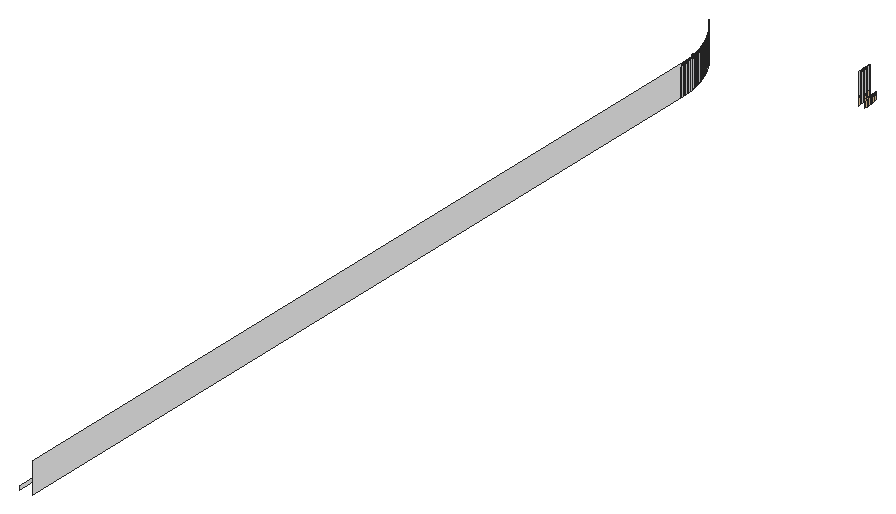
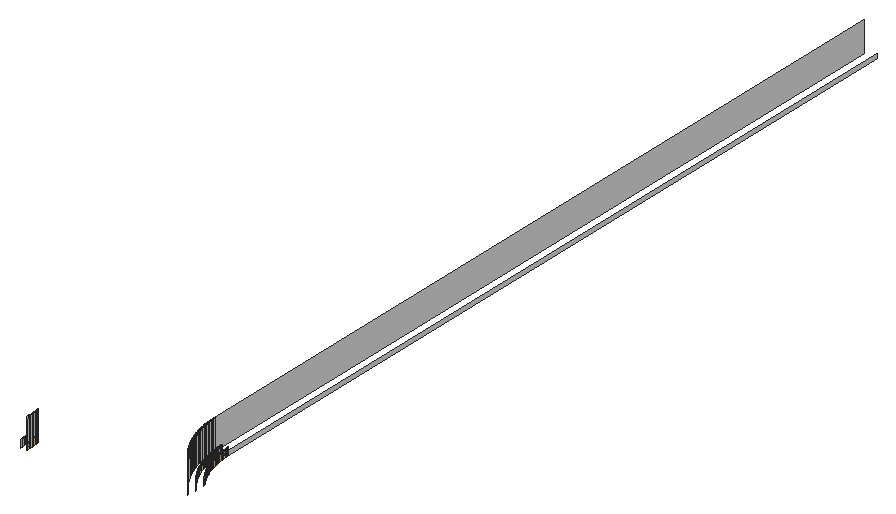
# SketchUp Ruby script. Lengths in inches.
U = 1.inch
M = Sketchup.active_model
def pt(a) = Geom::Point3d.new(a.map { |v| v * U })
def face(e, loops, mat)
  f = e.add_face(loops[0].map { |a| pt(a) })
  loops[1..].each { |l| e.add_face(l.map { |a| pt(a) }).erase! }
  f.material = f.back_material = mat if mat
  f
end
# faces: each face lists its corners as indices into pts; further lists are holes
def faces(e, pts, list, mat = nil) = list.each { |f| face(e, (f[0].is_a?(Array) ? f : [f]).map { |l| l.map { |i| pts[i] } }, mat) }
# xy, xz, yz: faces in a plane at the given z, y or x. An outline is a flat list of corners, or four numbers for a rectangle; further outlines are holes
def ring(l) = l.size == 4 ? [[l[0], l[1]], [l[2], l[1]], [l[2], l[3]], [l[0], l[3]]] : l.each_slice(2).to_a
def flat(e, list, mat, &to3) = list.each { |f| face(e, (f[0].is_a?(Array) ? f : [f]).map { |l| ring(l).map { |u, v| to3.(u, v) } }, mat) }
def xy(e, z, list, mat = nil) = flat(e, list, mat) { |x, y| [x, y, z] }
def xz(e, y, list, mat = nil) = flat(e, list, mat) { |x, z| [x, y, z] }
def yz(e, x, list, mat = nil) = flat(e, list, mat) { |y, z| [x, y, z] }
def lines(e, pts, list) = list.each { |a, b| e.add_line(pt(pts[a]), pt(pts[b])) }
# prism: a flat outline (further loops are holes) pulled along v
def prism(e, loops, v, mat = nil)
  f = face(e, loops, mat); d = Geom::Vector3d.new(v.map { |x| x * U })
  f.pushpull(f.normal.samedirection?(d) ? d.length : -d.length)
end
def box(e, o, s, mat = nil) = prism(e, [[o, [o[0] + s[0], o[1], o[2]], [o[0] + s[0], o[1] + s[1], o[2]], [o[0], o[1] + s[1], o[2]]]], [0, 0, s[2]], mat)
def at(x, y, z, deg = 0) = Geom::Transformation.translation(pt([x, y, z])) * Geom::Transformation.rotation(ORIGIN, Z_AXIS, deg.degrees)
def axes(o, x, y, z) = Geom::Transformation.new([*x, 0, *y, 0, *z, 0, *pt(o).to_a, 1])
def part(name) = M.definitions.add(name)
# library, detail: a bought-in or finely detailed component or shape, given as its bounding box
def library(name, o, s) = part(name).tap { |d| box(d.entities, o, s) }
def detail(e, o, s) = box(e.add_group.entities, o, s)
def put(e, d, t, mat = nil) = e.add_instance(d, t).tap { |i| i.material = mat if mat }
def group(e, t, mat = nil) = e.add_group.tap { |g| g.transformation = t; g.material = mat if mat }.entities
root = M.entities
M.materials.add("False Ceiling Light").color = [254, 223, 179]
M.materials.add("[Quartz Light Grey]").color = [251, 251, 252]
yz(root,178.5,[[204,115.32,204.18,116.49],[204.18,115.32,204.35,116.49]],"False Ceiling Light")
yz(root,178.5,[[78,115.32,204,115.91],[204,115.32,204.18,115.91],[204.18,115.32,204.35,115.91]],"[Quartz Light Grey]")
yz(root,179.5,[[204.01,115.32,204.19,116.49],[204.19,115.32,204.38,116.49]],"False Ceiling Light")
yz(root,180.49,[[204.41,115.32,204.61,120]],"[Quartz Light Grey]")
yz(root,180.5,[[77.99,115.32,204.01,120],[204.01,115.32,204.2,120]],"[Quartz Light Grey]")
yz(root,198.5,[[215.99,115.32,216.23,116.49],[216.23,115.32,216.45,116.49]],"False Ceiling Light")
yz(root,198.5,[[215.99,115.32,216.23,120],[216.23,115.32,216.45,120]],"[Quartz Light Grey]")
yz(root,199.5,[[216,115.32,216.24,116.49],[216.24,115.32,216.47,116.49]],"False Ceiling Light")
p = [[180.49,204.41,115.32],[180.5,204.2,115.32],[180.5,204.2,120],[180.49,204.41,120],[178.49,204.53,115.32],[178.5,204.35,115.32],
  [178.5,204.35,116.49],[178.49,204.53,116.49],[178.5,204.35,115.32],[178.49,204.53,115.32],[178.49,204.53,115.91],[178.5,204.35,115.91],
  [179.5,204.38,115.32],[179.49,204.57,115.32],[179.49,204.57,116.49],[179.5,204.38,116.49],[178.48,204.71,115.32],[178.48,204.71,116.49],
  [178.48,204.71,115.32],[178.48,204.71,115.91],[179.48,204.76,115.32],[179.48,204.76,116.49],[180.48,204.8125,115.32],[180.49,204.61,115.32],
  [180.49,204.61,120],[180.48,204.8125,120],[178.47,204.88,115.32],[178.47,204.88,116.49],[178.47,204.88,115.32],[178.47,204.88,115.91],
  [179.47,204.95,115.32],[179.47,204.95,116.49],[180.47,205.01,115.32],[180.47,205.01,120],[178.46,205.06,115.32],[178.46,205.06,116.49],
  [178.46,205.06,115.32],[178.46,205.06,115.91],[179.46,205.14,115.32],[179.46,205.14,116.49],[180.45,205.22,115.32],[180.45,205.22,120],
  [178.44,205.24,115.32],[178.44,205.24,116.49],[178.44,205.24,115.32],[178.44,205.24,115.91],[179.4375,205.33,115.32],[179.4375,205.33,116.49],
  [178.43,205.41,115.32],[178.43,205.41,116.49],[178.43,205.41,115.32],[178.43,205.41,115.91],[180.44,205.42,115.32],[180.44,205.42,120],
  [179.42,205.52,115.32],[179.42,205.52,116.49],[178.41,205.59,115.32],[178.41,205.59,116.49],[178.41,205.59,115.32],[178.41,205.59,115.91],
  [180.42,205.62,115.32],[180.42,205.62,120],[179.4,205.7,115.32],[179.4,205.7,116.49],[178.38,205.76,115.32],[178.38,205.76,116.49],
  [178.38,205.76,115.32],[178.38,205.76,115.91],[180.39,205.82,115.32],[180.39,205.82,120],[179.375,205.89,115.32],[179.375,205.89,116.49],
  [178.36,205.9375,115.32],[178.36,205.9375,116.49],[178.36,205.9375,115.32],[178.36,205.9375,115.91],[180.37,206.02,115.32],[180.37,206.02,120],
  [178.33,206.11,115.32],[178.33,206.11,116.49],[178.33,206.11,115.32],[178.33,206.11,115.91],[179.35,206.08,115.32],[179.35,206.08,116.49],
  [180.34,206.22,115.32],[180.34,206.22,120],[178.31,206.29,115.32],[178.31,206.29,116.49],[178.31,206.29,115.32],[178.31,206.29,115.91],
  [179.32,206.27,115.32],[179.32,206.27,116.49],[180.31,206.42,115.32],[180.31,206.42,120],[178.27,206.46,115.32],[178.27,206.46,116.49],
  [178.27,206.46,115.32],[178.27,206.46,115.91],[179.29,206.46,115.32],[179.29,206.46,116.49],[180.28,206.625,115.32],[180.28,206.625,120],
  [178.24,206.63,115.32],[178.24,206.63,116.49],[178.24,206.63,115.32],[178.24,206.63,115.91],[179.26,206.64,115.32],[179.26,206.64,116.49],
  [178.21,206.81,115.32],[178.21,206.81,116.49],[178.21,206.81,115.32],[178.21,206.81,115.91],[179.22,206.83,115.32],[179.22,206.83,116.49],
  [180.24,206.82,115.32],[180.24,206.82,120],[178.17,206.98,115.32],[178.17,206.98,116.49],[178.17,206.98,115.32],[178.17,206.98,115.91],
  [179.18,207.01,115.32],[179.18,207.01,116.49],[180.2,207.02,115.32],[180.2,207.02,120],[178.13,207.15,115.32],[178.13,207.15,116.49],
  [178.13,207.15,115.32],[178.13,207.15,115.91],[179.14,207.2,115.32],[179.14,207.2,116.49],[180.16,207.22,115.32],[180.16,207.22,120],
  [178.08,207.32,115.32],[178.08,207.32,116.49],[178.08,207.32,115.32],[178.08,207.32,115.91],[179.1,207.38,115.32],[179.1,207.38,116.49],
  [180.12,207.42,115.32],[180.12,207.42,120],[178.04,207.49,115.32],[178.04,207.49,116.49],[178.04,207.49,115.32],[178.04,207.49,115.91],
  [179.05,207.57,115.32],[179.05,207.57,116.49],[180.07,207.62,115.32],[180.07,207.62,120],[177.99,207.66,115.32],[177.99,207.66,116.49],
  [177.99,207.66,115.32],[177.99,207.66,115.91],[179.01,207.75,115.32],[179.01,207.75,116.49],[180.02,207.82,115.32],[180.02,207.82,120],
  [177.94,207.83,115.32],[177.94,207.83,116.49],[177.94,207.83,115.32],[177.94,207.83,115.91],[177.89,208,115.32],[177.89,208,116.49],
  [177.89,208,115.32],[177.89,208,115.91],[178.96,207.9375,115.32],[178.96,207.9375,116.49],[179.97,208.01,115.32],[179.97,208.01,120],
  [178.9,208.12,115.32],[178.9,208.12,116.49],[177.84,208.17,115.32],[177.84,208.17,116.49],[177.84,208.17,115.32],[177.84,208.17,115.91],
  [179.92,208.21,115.32],[179.92,208.21,120],[178.85,208.3,115.32],[178.85,208.3,116.49],[177.78,208.34,115.32],[177.78,208.34,116.49],
  [177.78,208.34,115.32],[177.78,208.34,115.91],[179.86,208.4,115.32],[179.86,208.4,120],[177.73,208.51,115.32],[177.73,208.51,116.49],
  [177.73,208.51,115.32],[177.73,208.51,115.91],[178.79,208.48,115.32],[178.79,208.48,116.49],[179.8,208.6,115.32],[179.8,208.6,120],
  [177.67,208.67,115.32],[177.67,208.67,116.49],[177.67,208.67,115.32],[177.67,208.67,115.91],[178.73,208.66,115.32],[178.73,208.66,116.49],
  [179.74,208.79,115.32],[179.74,208.79,120],[177.6,208.84,115.32],[177.6,208.84,116.49],[177.6,208.84,115.32],[177.6,208.84,115.91],
  [178.67,208.84,115.32],[178.67,208.84,116.49],[177.54,209,115.32],[177.54,209,116.49],[177.54,209,115.32],[177.54,209,115.91],
  [178.6,209.02,115.32],[178.6,209.02,116.49],[179.68,208.98,115.32],[179.68,208.98,120],[177.47,209.17,115.32],[177.47,209.17,116.49],
  [177.47,209.17,115.32],[177.47,209.17,115.91],[178.54,209.2,115.32],[178.54,209.2,116.49],[179.61,209.17,115.32],[179.61,209.17,120],
  [177.4,209.33,115.32],[177.4,209.33,116.49],[177.4,209.33,115.32],[177.4,209.33,115.91],[178.47,209.375,115.32],[178.47,209.375,116.49],
  [179.54,209.36,115.32],[179.54,209.36,120],[177.33,209.49,115.32],[177.33,209.49,116.49],[177.33,209.49,115.32],[177.33,209.49,115.91],
  [178.4,209.55,115.32],[178.4,209.55,116.49],[179.47,209.55,115.32],[179.47,209.55,120],[177.26,209.65,115.32],[177.26,209.65,116.49],
  [177.26,209.65,115.32],[177.26,209.65,115.91],[178.32,209.72,115.32],[178.32,209.72,116.49],[179.4,209.74,115.32],[179.4,209.74,120],
  [177.18,209.8125,115.32],[177.18,209.8125,116.49],[177.18,209.8125,115.32],[177.18,209.8125,115.91],[178.25,209.9,115.32],[178.25,209.9,116.49],
  [179.32,209.93,115.32],[179.32,209.93,120],[177.11,209.97,115.32],[177.11,209.97,116.49],[177.11,209.97,115.32],[177.11,209.97,115.91],
  [178.17,210.07,115.32],[178.17,210.07,116.49],[179.24,210.12,115.32],[179.24,210.12,120],[177.03,210.13,115.32],[177.03,210.13,116.49],
  [177.03,210.13,115.32],[177.03,210.13,115.91],[176.95,210.29,115.32],[176.95,210.29,116.49],[176.95,210.29,115.32],[176.95,210.29,115.91],
  [178.09,210.24,115.32],[178.09,210.24,116.49],[179.16,210.3,115.32],[179.16,210.3,120],[178,210.41,115.32],[178,210.41,116.49],
  [176.86,210.44,115.32],[176.86,210.44,116.49],[176.86,210.44,115.32],[176.86,210.44,115.91],[179.08,210.49,115.32],[179.08,210.49,120],
  [176.78,210.6,115.32],[176.78,210.6,116.49],[176.78,210.6,115.32],[176.78,210.6,115.91],[177.92,210.58,115.32],[177.92,210.58,116.49],
  [178.99,210.67,115.32],[178.99,210.67,120],[176.69,210.75,115.32],[176.69,210.75,116.49],[176.69,210.75,115.32],[176.69,210.75,115.91],
  [177.83,210.75,115.32],[177.83,210.75,116.49],[178.9,210.86,115.32],[178.9,210.86,120],[176.6,210.9,115.32],[176.6,210.9,116.49],
  [176.6,210.9,115.32],[176.6,210.9,115.91],[177.74,210.92,115.32],[177.74,210.92,116.49],[176.51,211.05,115.32],[176.51,211.05,116.49],
  [176.51,211.05,115.32],[176.51,211.05,115.91],[177.65,211.09,115.32],[177.65,211.09,116.49],[178.8125,211.04,115.32],[178.8125,211.04,120],
  [178.72,211.22,115.32],[178.72,211.22,120],[176.42,211.2,115.32],[176.42,211.2,116.49],[176.42,211.2,115.32],[176.42,211.2,115.91],
  [177.56,211.25,115.32],[177.56,211.25,116.49],[176.32,211.35,115.32],[176.32,211.35,116.49],[176.32,211.35,115.32],[176.32,211.35,115.91],
  [178.62,211.4,115.32],[178.62,211.4,120],[177.46,211.41,115.32],[177.46,211.41,116.49],[176.22,211.5,115.32],[176.22,211.5,116.49],
  [176.22,211.5,115.32],[176.22,211.5,115.91],[177.36,211.58,115.32],[177.36,211.58,116.49],[178.52,211.57,115.32],[178.52,211.57,120],
  [176.125,211.65,115.32],[176.125,211.65,116.49],[176.125,211.65,115.32],[176.125,211.65,115.91],[177.26,211.74,115.32],[177.26,211.74,116.49],
  [178.42,211.75,115.32],[178.42,211.75,120],[177.16,211.9,115.32],[177.16,211.9,116.49],[178.32,211.93,115.32],[178.32,211.93,120],
  [177.06,212.06,115.32],[177.06,212.06,116.49],[178.22,212.1,115.32],[178.22,212.1,120],[176.95,212.21,115.32],[176.95,212.21,116.49],
  [178.11,212.27,115.32],[178.11,212.27,120],[176.84,212.37,115.32],[176.84,212.37,116.49],[178,212.44,115.32],[178,212.44,120],
  [176.73,212.52,115.32],[176.73,212.52,116.49],[177.89,212.61,115.32],[177.89,212.61,120],[176.62,212.68,115.32],[176.62,212.68,116.49],
  [177.77,212.78,115.32],[177.77,212.78,120],[176.5,212.83,115.32],[176.5,212.83,116.49],[176.39,212.98,115.32],[176.39,212.98,116.49],
  [177.66,212.95,115.32],[177.66,212.95,120],[177.54,213.11,115.32],[177.54,213.11,120],[176.27,213.125,115.32],[176.27,213.125,116.49],
  [176.15,213.27,115.32],[176.15,213.27,116.49],[177.42,213.27,115.32],[177.42,213.27,120],[177.3,213.4375,115.32],[177.3,213.4375,120],
  [177.17,213.6,115.32],[177.17,213.6,120],[177.05,213.75,115.32],[177.05,213.75,120],[176.92,213.91,115.32],[176.92,213.91,120],
  [176.79,214.07,115.32],[176.79,214.07,120],[176.65,214.22,115.32],[176.65,214.22,120],[176.52,214.37,115.32],[176.52,214.37,120],
  [176.38,214.52,115.32],[176.38,214.52,120],[176.24,214.67,115.32],[176.24,214.67,120],[198.5,216.45,115.32],[198.49,216.68,115.32],
  [198.49,216.68,120],[198.5,216.45,120],[198.49,216.68,115.32],[198.5,216.45,115.32],[198.5,216.45,116.49],[198.49,216.68,116.49],
  [199.5,216.47,115.32],[199.49,216.71,115.32],[199.49,216.71,116.49],[199.5,216.47,116.49],[198.48,216.9,115.32],[198.48,216.9,120],
  [198.48,216.9,115.32],[198.48,216.9,116.49],[199.48,216.94,115.32],[199.48,216.94,116.49],[198.47,217.125,115.32],[198.47,217.125,120],
  [198.47,217.125,115.32],[198.47,217.125,116.49],[199.47,217.18,115.32],[199.47,217.18,116.49],[198.46,217.35,115.32],[198.46,217.35,120],
  [198.46,217.35,115.32],[198.46,217.35,116.49],[199.46,217.41,115.32],[199.46,217.41,116.49],[198.44,217.57,115.32],[198.44,217.57,120],
  [198.44,217.57,115.32],[198.44,217.57,116.49],[199.44,217.65,115.32],[199.44,217.65,116.49],[198.42,217.8,115.32],[198.42,217.8,120],
  [198.42,217.8,115.32],[198.42,217.8,116.49],[199.42,217.88,115.32],[199.42,217.88,116.49],[198.4,218.02,115.32],[198.4,218.02,120],
  [198.4,218.02,115.32],[198.4,218.02,116.49],[199.4,218.12,115.32],[199.4,218.12,116.49],[198.38,218.25,115.32],[198.38,218.25,120],
  [198.38,218.25,115.32],[198.38,218.25,116.49],[199.375,218.35,115.32],[199.375,218.35,116.49],[176.9375,216,120],[177,216,120],
  [177,215.9375,120]]
faces(root,p,[[0,1,2,3],[8,9,10,11],[9,18,19,10],[22,23,24,25],[18,28,29,19],[32,22,25,33],[28,36,37,29],[40,32,33,41],
  [36,44,45,37],[44,50,51,45],[52,40,41,53],[50,58,59,51],[60,52,53,61],[58,66,67,59],[68,60,61,69],[66,74,75,67],
  [76,68,69,77],[74,80,81,75],[84,76,77,85],[80,88,89,81],[92,84,85,93],[88,96,97,89],[100,92,93,101],[96,104,105,97],
  [104,110,111,105],[114,100,101,115],[110,118,119,111],[122,114,115,123],[118,126,127,119],[130,122,123,131],[126,134,135,127],[138,130,131,139],
  [134,142,143,135],[146,138,139,147],[142,150,151,143],[154,146,147,155],[150,158,159,151],[158,162,163,159],[166,154,155,167],[162,172,173,163],
  [174,166,167,175],[172,180,181,173],[182,174,175,183],[180,186,187,181],[190,182,183,191],[186,194,195,187],[198,190,191,199],[194,202,203,195],
  [202,208,209,203],[212,198,199,213],[208,216,217,209],[220,212,213,221],[216,224,225,217],[228,220,221,229],[224,232,233,225],[236,228,229,237],
  [232,240,241,233],[244,236,237,245],[240,248,249,241],[252,244,245,253],[248,256,257,249],[260,252,253,261],[256,264,265,257],[264,268,269,265],
  [272,260,261,273],[268,278,279,269],[280,272,273,281],[278,284,285,279],[288,280,281,289],[284,292,293,285],[296,288,289,297],[292,300,301,293],
  [300,306,307,301],[310,296,297,311],[312,310,311,313],[306,316,317,307],[316,322,323,317],[324,312,313,325],[322,330,331,323],[334,324,325,335],
  [330,338,339,331],[342,334,335,343],[346,342,343,347],[350,346,347,351],[354,350,351,355],[358,354,355,359],[362,358,359,363],[366,362,363,367],
  [372,366,367,373],[374,372,373,375],[380,374,375,381],[382,380,381,383],[384,382,383,385],[386,384,385,387],[388,386,387,389],[390,388,389,391],
  [392,390,391,393],[394,392,393,395],[396,394,395,397],[398,396,397,399],[400,401,402,403],[401,412,413,402],[412,418,419,413],[418,424,425,419],
  [424,430,431,425],[430,436,437,431],[436,442,443,437],[442,448,449,443]],"[Quartz Light Grey]")
faces(root,p,[[4,5,6,7],[12,13,14,15],[16,4,7,17],[13,20,21,14],[26,16,17,27],[20,30,31,21],[34,26,27,35],[30,38,39,31],
  [42,34,35,43],[38,46,47,39],[48,42,43,49],[46,54,55,47],[56,48,49,57],[54,62,63,55],[64,56,57,65],[62,70,71,63],
  [72,64,65,73],[78,72,73,79],[70,82,83,71],[86,78,79,87],[82,90,91,83],[94,86,87,95],[90,98,99,91],[102,94,95,103],
  [98,106,107,99],[108,102,103,109],[106,112,113,107],[116,108,109,117],[112,120,121,113],[124,116,117,125],[120,128,129,121],[132,124,125,133],
  [128,136,137,129],[140,132,133,141],[136,144,145,137],[148,140,141,149],[144,152,153,145],[156,148,149,157],[160,156,157,161],[152,164,165,153],
  [164,168,169,165],[170,160,161,171],[168,176,177,169],[178,170,171,179],[184,178,179,185],[176,188,189,177],[192,184,185,193],[188,196,197,189],
  [200,192,193,201],[196,204,205,197],[206,200,201,207],[204,210,211,205],[214,206,207,215],[210,218,219,211],[222,214,215,223],[218,226,227,219],
  [230,222,223,231],[226,234,235,227],[238,230,231,239],[234,242,243,235],[246,238,239,247],[242,250,251,243],[254,246,247,255],[250,258,259,251],
  [262,254,255,263],[266,262,263,267],[258,270,271,259],[270,274,275,271],[276,266,267,277],[282,276,277,283],[274,286,287,275],[290,282,283,291],
  [286,294,295,287],[298,290,291,299],[294,302,303,295],[304,298,299,305],[302,308,309,303],[314,304,305,315],[308,318,319,309],[320,314,315,321],
  [318,326,327,319],[328,320,321,329],[326,332,333,327],[336,328,329,337],[332,340,341,333],[340,344,345,341],[344,348,349,345],[348,352,353,349],
  [352,356,357,353],[356,360,361,357],[360,364,365,361],[364,368,369,365],[368,370,371,369],[370,376,377,371],[376,378,379,377],[404,405,406,407],
  [408,409,410,411],[414,404,407,415],[409,416,417,410],[420,414,415,421],[416,422,423,417],[426,420,421,427],[422,428,429,423],[432,426,427,433],
  [428,434,435,429],[438,432,433,439],[434,440,441,435],[444,438,439,445],[440,446,447,441],[450,444,445,451],[446,452,453,447]],"False Ceiling Light")
lines(root,p,[[454,455],[455,456]])
